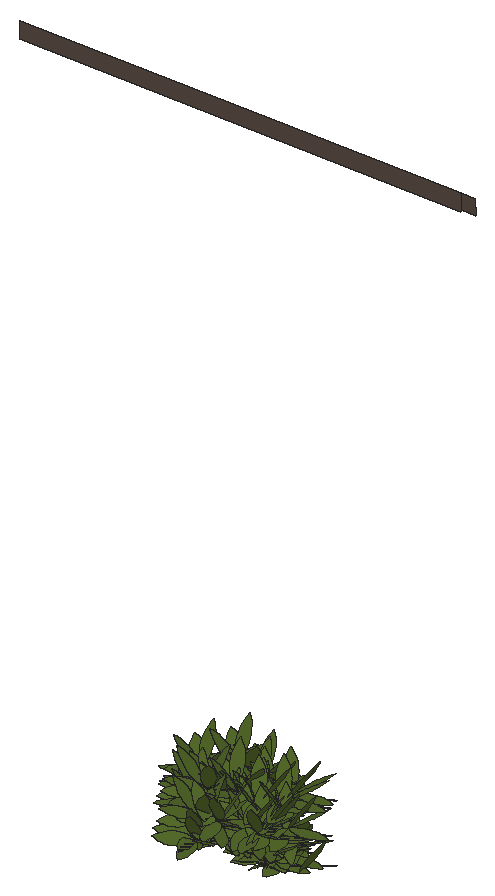
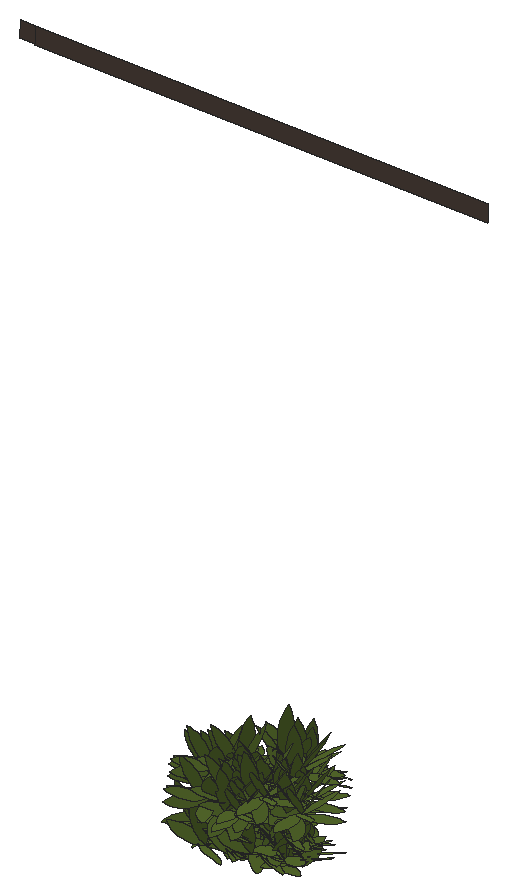
# SketchUp Ruby script. Lengths in inches.
U = 1.inch
M = Sketchup.active_model
def pt(a) = Geom::Point3d.new(a.map { |v| v * U })
def face(e, loops, mat)
  f = e.add_face(loops[0].map { |a| pt(a) })
  loops[1..].each { |l| e.add_face(l.map { |a| pt(a) }).erase! }
  f.material = f.back_material = mat if mat
  f
end
# faces: each face lists its corners as indices into pts; further lists are holes
def faces(e, pts, list, mat = nil) = list.each { |f| face(e, (f[0].is_a?(Array) ? f : [f]).map { |l| l.map { |i| pts[i] } }, mat) }
# xy, xz, yz: faces in a plane at the given z, y or x. An outline is a flat list of corners, or four numbers for a rectangle; further outlines are holes
def ring(l) = l.size == 4 ? [[l[0], l[1]], [l[2], l[1]], [l[2], l[3]], [l[0], l[3]]] : l.each_slice(2).to_a
def flat(e, list, mat, &to3) = list.each { |f| face(e, (f[0].is_a?(Array) ? f : [f]).map { |l| ring(l).map { |u, v| to3.(u, v) } }, mat) }
def xy(e, z, list, mat = nil) = flat(e, list, mat) { |x, y| [x, y, z] }
def xz(e, y, list, mat = nil) = flat(e, list, mat) { |x, z| [x, y, z] }
def yz(e, x, list, mat = nil) = flat(e, list, mat) { |y, z| [x, y, z] }
def lines(e, pts, list) = list.each { |a, b| e.add_line(pt(pts[a]), pt(pts[b])) }
# prism: a flat outline (further loops are holes) pulled along v
def prism(e, loops, v, mat = nil)
  f = face(e, loops, mat); d = Geom::Vector3d.new(v.map { |x| x * U })
  f.pushpull(f.normal.samedirection?(d) ? d.length : -d.length)
end
def box(e, o, s, mat = nil) = prism(e, [[o, [o[0] + s[0], o[1], o[2]], [o[0] + s[0], o[1] + s[1], o[2]], [o[0], o[1] + s[1], o[2]]]], [0, 0, s[2]], mat)
def at(x, y, z, deg = 0) = Geom::Transformation.translation(pt([x, y, z])) * Geom::Transformation.rotation(ORIGIN, Z_AXIS, deg.degrees)
def axes(o, x, y, z) = Geom::Transformation.new([*x, 0, *y, 0, *z, 0, *pt(o).to_a, 1])
def part(name) = M.definitions.add(name)
# library, detail: a bought-in or finely detailed component or shape, given as its bounding box
def library(name, o, s) = part(name).tap { |d| box(d.entities, o, s) }
def detail(e, o, s) = box(e.add_group.entities, o, s)
def put(e, d, t, mat = nil) = e.add_instance(d, t).tap { |i| i.material = mat if mat }
def group(e, t, mat = nil) = e.add_group.tap { |g| g.transformation = t; g.material = mat if mat }.entities
root = M.entities
M.materials.add("2").color = [91, 76, 69]
M.materials.add("[Asphalt_New]").color = [85, 106, 44]
M.materials.add("white").color = [255, 255, 255]
c1 = part("Component\#59")
xy(c1.entities,0,[[5.79,0,4.75,0.06,3.73,0.22,2.73,0.5,1.77,0.88,0.86,1.37,0,1.95,0.83,2.59,1.74,3.13,2.7,3.56,3.7,3.87,4.74,4.05,5.79,4.12,6.84,4.05,7.87,3.87,8.88,3.56,9.84,3.13,10.74,2.59,11.57,1.95,10.72,1.37,9.8,0.88,8.84,0.5,7.84,0.22,6.82,0.06]],"[Asphalt_New]")
c2 = part("Leaf cluster")
put(c2.entities,c1,axes([10.37,9.23,1.73],[-0.67725,-0.67301,0.29729],[0.61625,-0.73963,-0.27052],[0.40195,0,0.91566]),"[Asphalt_New]")
put(c2.entities,c1,at(0,5.84,1.2),"[Asphalt_New]")
put(c2.entities,c1,axes([11.625,9.72,1.52],[-0.61694,-0.11161,0.77906],[-0.02647,-0.98639,-0.16227],[0.78657,-0.12073,0.60559]),"[Asphalt_New]")
put(c2.entities,c1,axes([13.35,8.05,1.98],[-0.1211,0.99122,-0.05316],[-0.90762,-0.13226,-0.39842],[-0.40195,0,0.91566]),"[Asphalt_New]")
c3 = part("Groupe\#6")
put(c3.entities,c2,axes([6.2,8.72,2.56],[0.20072,0.20931,0],[-0.20931,0.20072,0],[0,0,0.3393]))
put(c3.entities,c2,axes([3.21,14.77,2.82],[0.12393,-0.26218,0],[0.26218,0.12393,0],[0,0,0.3393]))
put(c3.entities,c1,axes([6.98,12.58,2.74],[0.18147,-0.01125,0.26433],[0.07569,0.27597,-0.05506],[-0.21317,0.08841,0.20548]),"[Asphalt_New]")
put(c3.entities,c2,axes([9.62,7.71,2.12],[0.13301,0.2577,0],[-0.2577,0.13301,0],[0,0,0.3393]))
put(c3.entities,c2,axes([5.04,12.65,2.375],[0.19329,-0.21619,0],[0.21619,0.19329,0],[0,0,0.3393]))
put(c3.entities,c2,axes([8.55,8.27,2.12],[0.13301,0.2577,0],[-0.2577,0.13301,0],[0,0,0.3393]))
put(c3.entities,c2,axes([3.97,13.21,2.375],[0.19329,-0.21619,0],[0.21619,0.19329,0],[0,0,0.3393]))
put(c3.entities,c2,axes([13.2,6.93,2.95],[-0.24238,0.15922,0],[-0.15922,-0.24238,0],[0,0,0.3393]))
put(c3.entities,c2,axes([7.8,2.89,3.21],[0.23521,0.16964,0],[-0.16964,0.23521,0],[0,0,0.3393]))
put(c3.entities,c1,axes([9.26,7,3.13],[-0.02201,0.18048,0.26433],[-0.28514,0.02413,-0.05506],[-0.04808,-0.22571,0.20548]),"[Asphalt_New]")
put(c3.entities,c2,axes([10.92,8.49,3.88],[-0.24238,0.15922,0],[-0.15922,-0.24238,0],[0,0,0.3393]))
put(c3.entities,c2,axes([5.52,4.45,4.14],[0.23521,0.16964,0],[-0.16964,0.23521,0],[0,0,0.3393]))
put(c3.entities,c1,axes([6.97,8.56,4.0625],[-0.02201,0.18048,0.26433],[-0.28514,0.02413,-0.05506],[-0.04808,-0.22571,0.20548]),"[Asphalt_New]")
put(c3.entities,c2,axes([9.9,10.06,2.52],[-0.24238,0.15922,0],[-0.15922,-0.24238,0],[0,0,0.3393]))
put(c3.entities,c2,axes([4.51,6.02,2.78],[0.23521,0.16964,0],[-0.16964,0.23521,0],[0,0,0.3393]))
put(c3.entities,c1,axes([5.96,10.125,2.71],[-0.02201,0.18048,0.26433],[-0.28514,0.02413,-0.05506],[-0.04808,-0.22571,0.20548]),"[Asphalt_New]")
put(c3.entities,c2,axes([13.6,14.86,2.41],[-0.24779,-0.15066,0],[0.15066,-0.24779,0],[0,0,0.3393]))
put(c3.entities,c2,axes([8.65,12.2,2.15],[0.22914,-0.17774,0],[0.17774,0.22914,0],[0,0,0.3393]))
put(c3.entities,c2,axes([14.35,15.81,2.41],[-0.24779,-0.15066,0],[0.15066,-0.24779,0],[0,0,0.3393]))
put(c3.entities,c2,axes([7.9,11.25,2.15],[0.22914,-0.17774,0],[0.17774,0.22914,0],[0,0,0.3393]))
put(c3.entities,c2,axes([-0.46,12.1,3.24],[0.12393,-0.26218,0],[0.26218,0.12393,0],[0,0,0.3393]))
put(c3.entities,c1,axes([3.31,9.91,3.17],[0.18147,-0.01125,0.26433],[0.07569,0.27597,-0.05506],[-0.21317,0.08841,0.20548]),"[Asphalt_New]")
put(c3.entities,c2,axes([4.47,8.01,3.91],[0.20072,0.20931,0],[-0.20931,0.20072,0],[0,0,0.3393]))
put(c3.entities,c2,axes([1.49,14.06,4.17],[0.12393,-0.26218,0],[0.26218,0.12393,0],[0,0,0.3393]))
put(c3.entities,c1,axes([5.26,11.88,4.1],[0.18147,-0.01125,0.26433],[0.07569,0.27597,-0.05506],[-0.21317,0.08841,0.20548]),"[Asphalt_New]")
put(c3.entities,c2,axes([6.85,4.1,2.54],[0.13301,0.2577,0],[-0.2577,0.13301,0],[0,0,0.3393]))
put(c3.entities,c2,axes([2.27,9.05,2.8],[0.19329,-0.21619,0],[0.21619,0.19329,0],[0,0,0.3393]))
put(c3.entities,c1,axes([6.51,8.03,2.73],[0.17719,0.04076,0.26433],[-0.00581,0.2861,-0.05506],[-0.2295,0.02423,0.20548]),"[Asphalt_New]")
put(c3.entities,c2,axes([4.86,14.63,2.58],[0.22914,-0.17774,0],[0.17774,0.22914,0],[0,0,0.3393]))
put(c3.entities,c2,axes([10.5625,18.23,2.83],[-0.24779,-0.15066,0],[0.15066,-0.24779,0],[0,0,0.3393]))
put(c3.entities,c1,axes([8.79,14.25,2.76],[0.00779,-0.18165,0.26433],[0.28237,-0.04643,-0.05506],[0.06564,0.22124,0.20548]),"[Asphalt_New]")
put(c3.entities,c2,axes([7.02,12.9,3.51],[0.22914,-0.17774,0],[0.17774,0.22914,0],[0,0,0.3393]))
put(c3.entities,c2,axes([12.72,16.5,3.76],[-0.24779,-0.15066,0],[0.15066,-0.24779,0],[0,0,0.3393]))
put(c3.entities,c1,axes([10.94,12.52,3.6875],[0.00779,-0.18165,0.26433],[0.28237,-0.04643,-0.05506],[0.06564,0.22124,0.20548]),"[Asphalt_New]")
put(c3.entities,c2,axes([5.98,10.15,2.19],[0.23521,0.16964,0],[-0.16964,0.23521,0],[0,0,0.3393]))
put(c3.entities,c2,axes([9.23,9.05,2.52],[-0.24238,0.15922,0],[-0.15922,-0.24238,0],[0,0,0.3393]))
put(c3.entities,c2,axes([3.84,5.01,2.78],[0.23521,0.16964,0],[-0.16964,0.23521,0],[0,0,0.3393]))
put(c3.entities,c1,axes([5.29,9.12,2.71],[-0.02201,0.18048,0.26433],[-0.28514,0.02413,-0.05506],[-0.04808,-0.22571,0.20548]),"[Asphalt_New]")
put(c3.entities,c2,axes([4.09,12.81,2.58],[0.23461,-0.17046,0],[0.17046,0.23461,0],[0,0,0.3393]))
put(c3.entities,c2,axes([9.68,16.59,2.83],[-0.24294,-0.15837,0],[0.15837,-0.24294,0],[0,0,0.3393]))
put(c3.entities,c1,axes([8.03,12.56,2.76],[0.01349,-0.18132,0.26433],[0.28368,-0.03753,-0.05506],[0.05866,0.22319,0.20548]),"[Asphalt_New]")
put(c3.entities,c2,axes([6.3,11.15,3.51],[0.23461,-0.17046,0],[0.17046,0.23461,0],[0,0,0.3393]))
put(c3.entities,c2,axes([11.89,14.93,3.76],[-0.24294,-0.15837,0],[0.15837,-0.24294,0],[0,0,0.3393]))
put(c3.entities,c1,axes([10.24,10.89,3.6875],[0.01349,-0.18132,0.26433],[0.28368,-0.03753,-0.05506],[0.05866,0.22319,0.20548]),"[Asphalt_New]")
put(c3.entities,c2,axes([11.75,13.77,2.17],[-0.145,-0.25115,0],[0.25115,-0.145,0],[0,0,0.3393]))
put(c3.entities,c2,axes([16.09,8.62,2.43],[-0.1829,0.22505,0],[-0.22505,-0.1829,0],[0,0,0.3393]))
put(c3.entities,c2,axes([10.33,11.4,3.1],[-0.145,-0.25115,0],[0.25115,-0.145,0],[0,0,0.3393]))
put(c3.entities,c2,axes([14.67,6.25,3.36],[-0.1829,0.22505,0],[-0.22505,-0.1829,0],[0,0,0.3393]))
put(c3.entities,c1,axes([10.48,7.46,3.28],[-0.17891,-0.03237,0.26433],[-0.00768,-0.28605,-0.05506],[0.2281,-0.03501,0.20548]),"[Asphalt_New]")
put(c3.entities,c2,axes([7.24,9.53,2.15],[0.23461,-0.17046,0],[0.17046,0.23461,0],[0,0,0.3393]))
put(c3.entities,c2,axes([12.82,13.3125,2.41],[-0.24294,-0.15837,0],[0.15837,-0.24294,0],[0,0,0.3393]))
put(c3.entities,c2,axes([7.96,10.51,2.15],[0.23461,-0.17046,0],[0.17046,0.23461,0],[0,0,0.3393]))
put(c3.entities,c2,axes([13.54,14.29,2.41],[-0.24294,-0.15837,0],[0.15837,-0.24294,0],[0,0,0.3393]))
put(c3.entities,c2,axes([10,6.52,1.96],[0.20072,0.20931,0],[-0.20931,0.20072,0],[0,0,0.3393]))
put(c3.entities,c2,axes([7.01,12.5625,2.22],[0.12393,-0.26218,0],[0.26218,0.12393,0],[0,0,0.3393]))
put(c3.entities,c2,axes([5.33,9.5625,2.56],[0.20072,0.20931,0],[-0.20931,0.20072,0],[0,0,0.3393]))
put(c3.entities,c2,axes([2.34,15.61,2.82],[0.12393,-0.26218,0],[0.26218,0.12393,0],[0,0,0.3393]))
put(c3.entities,c1,axes([6.12,13.43,2.74],[0.18147,-0.01125,0.26433],[0.07569,0.27597,-0.05506],[-0.21317,0.08841,0.20548]),"[Asphalt_New]")
put(c3.entities,c2,axes([13.16,5.15,2],[-0.1829,0.22505,0],[-0.22505,-0.1829,0],[0,0,0.3393]))
put(c3.entities,c2,axes([14.2,4.53,2],[-0.1829,0.22505,0],[-0.22505,-0.1829,0],[0,0,0.3393]))
put(c3.entities,c2,axes([8.17,6.54,3.47],[0.13301,0.2577,0],[-0.2577,0.13301,0],[0,0,0.3393]))
put(c3.entities,c2,axes([3.58,11.48,3.73],[0.19329,-0.21619,0],[0.21619,0.19329,0],[0,0,0.3393]))
put(c3.entities,c1,axes([7.82,10.46,3.66],[0.17719,0.04076,0.26433],[-0.00581,0.2861,-0.05506],[-0.2295,0.02423,0.20548]),"[Asphalt_New]")
put(c3.entities,c2,axes([2.52,6.05,2.98],[0.20072,0.20931,0],[-0.20931,0.20072,0],[0,0,0.3393]))
xz(root,18.35,[[127.1875,121.625,148.875,122.4375]],"2")
p = [[148.875,18.37,121.69],[148.875,18.35,122.4375],[149.5625,18.35,122.4375],[149.5625,18.37,121.69]]
faces(root,p,[[0,1,2,3]],"2")
put(root,c2,axes([137.9,16.39,91.26],[0.1271,-0.08349,0],[0.08349,0.1271,0],[0,0,0.17792]),"white")
put(root,c2,axes([140.13,17.43,90.54],[-0.12016,0.09321,0],[-0.09321,-0.12016,0],[0,0,0.17792]),"white")
put(root,c2,axes([138.78,17.14,90.66],[-0.10136,0.11337,0],[-0.11337,-0.10136,0],[0,0,0.17792]),"white")
put(root,c3,axes([132.83,13.8,90.97],[0.48162,-0.20742,0],[0.20742,0.48162,0],[0,0,0.52438]),"white")
put(root,c1,axes([139.62,16.72,90.71],[0.15184,-0.00221,-0.00946],[-0.00119,0.13948,-0.07089],[0.0083,0.06056,0.16292]),"[Asphalt_New]")
put(root,c1,axes([138.09,16.1,90.93],[0.01807,0.15078,-0.00946],[-0.13884,0.01339,-0.07089],[-0.05936,0.01458,0.16292]),"[Asphalt_New]")
put(root,c1,axes([139.68,17.45,91.36],[-0.09292,-0.02137,0.13861],[0.00305,-0.15002,-0.02887],[0.12035,-0.0127,0.10775]),"[Asphalt_New]")
put(root,c1,axes([140.15,16.21,90.46],[0.10299,0.10235,0.0529],[-0.09371,0.11248,-0.04813],[-0.06112,0,0.16292]),"[Asphalt_New]")
put(root,c1,axes([137.5625,16.64,90.39],[0.09382,0.01697,0.13861],[0.00402,0.15,-0.02887],[-0.11961,0.01836,0.10775]),"[Asphalt_New]")
put(root,c1,axes([141.55,16.16,91.68],[0.01807,0.15078,-0.00946],[-0.13884,0.01339,-0.07089],[-0.05936,0.01458,0.16292]),"[Asphalt_New]")
put(root,c1,axes([139.71,17.42,92.15],[-0.15155,-0.00971,-0.00946],[0.01213,-0.13895,-0.07089],[-0.00352,-0.06102,0.16292]),"[Asphalt_New]")
put(root,c1,axes([138.73,16.19,91.52],[0.00875,0.15182,0],[-0.15182,0.00875,0],[0,0,0.17792]),"[Asphalt_New]")
put(root,c1,axes([140.83,16.19,90.9],[0.01807,0.15078,-0.00946],[-0.13884,0.01339,-0.07089],[-0.05936,0.01458,0.16292]),"[Asphalt_New]")
put(root,c1,axes([140.34,17.93,90.71],[0.01842,-0.15074,-0.00946],[0.13802,0.02011,-0.07089],[0.06112,0,0.16292]),"[Asphalt_New]")
put(root,c1,axes([137.94,16.78,91.31],[0.1519,0.00716,0],[-0.00716,0.1519,0],[0,0,0.17792]),"[Asphalt_New]")
put(root,c2,axes([139.35,16.82,90.89],[-0.06499,0.13748,0],[-0.13748,-0.06499,0],[0,0,0.17792]),"white")
put(root,c1,axes([137.34,18,91.74],[0.01842,-0.15074,-0.00946],[0.13802,0.02011,-0.07089],[0.06112,0,0.16292]),"[Asphalt_New]")
put(root,c2,axes([140.68,15.61,90.54],[0.07604,0.1317,0],[-0.1317,0.07604,0],[0,0,0.17792]),"white")
put(root,c1,axes([138.6,17.52,90.89],[-0.15155,-0.00971,-0.00946],[0.01213,-0.13895,-0.07089],[-0.00352,-0.06102,0.16292]),"[Asphalt_New]")
put(root,c1,axes([136.46,18.11,91.1],[-0.0159,-0.15124,0],[0.15124,-0.0159,0],[0,0,0.17792]),"[Asphalt_New]")
put(root,c2,axes([137.14,15.54,90.67],[0.12994,0.079,0],[-0.079,0.12994,0],[0,0,0.17792]),"white")
put(root,c1,axes([137.17,17.94,90.88],[-0.12443,-0.07482,0.0529],[0.06418,-0.13158,-0.04813],[0.05936,-0.01458,0.16292]),"[Asphalt_New]")
put(root,c2,axes([142.28,17.75,90.54],[-0.12303,0.08939,0],[-0.08939,-0.12303,0],[0,0,0.17792]),"white")
put(root,c2,axes([137.68,15.68,91.56],[0.07604,0.1317,0],[-0.1317,0.07604,0],[0,0,0.17792]),"white")
put(root,c2,axes([136.99,18.93,90.75],[-0.10525,-0.10976,0],[0.10976,-0.10525,0],[0,0,0.17792]),"white")
put(root,c1,axes([138.99,17,90.71],[0.15184,-0.00221,-0.00946],[-0.00119,0.13948,-0.07089],[0.0083,0.06056,0.16292]),"[Asphalt_New]")
put(root,c1,axes([138.43,17.5625,90.85],[-0.09516,0.0059,0.13861],[-0.03969,-0.14471,-0.02887],[0.11178,-0.04636,0.10775]),"[Asphalt_New]")
put(root,c2,axes([142.13,17.77,90.32],[-0.12016,0.09321,0],[-0.09321,-0.12016,0],[0,0,0.17792]),"white")
put(root,c2,axes([141.08,19.04,91.39],[-0.12334,-0.08896,0],[0.08896,-0.12334,0],[0,0,0.17792]),"white")
put(root,c1,axes([138.3,17.8,91.61],[0.09625,-0.10871,0.0529],[0.11768,0.08708,-0.04813],[0.00352,0.06102,0.16292]),"[Asphalt_New]")
put(root,c2,axes([135.37,17.28,90.43],[0.09591,-0.11801,0],[0.11801,0.09591,0],[0,0,0.17792]),"white")
put(root,c2,axes([140.74,17.02,90.89],[-0.06499,0.13748,0],[-0.13748,-0.06499,0],[0,0,0.17792]),"white")
put(root,c1,axes([137.24,16.8,91.16],[-0.00707,0.09508,0.13861],[-0.14876,0.01968,-0.02887],[-0.03076,-0.11704,0.10775]),"[Asphalt_New]")
put(root,c1,axes([137.04,16.58,91.2],[0.10299,0.10235,0.0529],[-0.09371,0.11248,-0.04813],[-0.06112,0,0.16292]),"[Asphalt_New]")
put(root,c2,axes([139.89,17.86,90.75],[-0.12016,0.09321,0],[-0.09321,-0.12016,0],[0,0,0.17792]),"white")
put(root,c1,axes([138.24,17.99,91.58],[0.01154,-0.09464,0.13861],[0.14952,-0.01265,-0.02887],[0.02521,0.11836,0.10775]),"[Asphalt_New]")
put(root,c1,axes([138.5625,18.14,90.88],[-0.12443,-0.07482,0.0529],[0.06418,-0.13158,-0.04813],[0.05936,-0.01458,0.16292]),"[Asphalt_New]")
put(root,c2,axes([139.35,15.77,90.67],[0.12739,0.08305,0],[-0.08305,0.12739,0],[0,0,0.17792]),"white")
put(root,c1,axes([136.77,16.59,90.93],[0.01807,0.15078,-0.00946],[-0.13884,0.01339,-0.07089],[-0.05936,0.01458,0.16292]),"[Asphalt_New]")
put(root,c2,axes([141.64,18,90.54],[-0.12303,0.08939,0],[-0.08939,-0.12303,0],[0,0,0.17792]),"white")
put(root,c2,axes([138.25,16.92,91.26],[0.1271,-0.08349,0],[0.08349,0.1271,0],[0,0,0.17792]),"white")
put(root,c1,axes([136.57,17.41,90.79],[0.14768,-0.03627,0],[0.03627,0.14768,0],[0,0,0.17792]),"[Asphalt_New]")
put(root,c1,axes([137.75,16.72,90.43],[0.10299,0.10235,0.0529],[-0.09371,0.11248,-0.04813],[-0.06112,0,0.16292]),"[Asphalt_New]")
put(root,c1,axes([139.91,16.95,90.63],[-0.00408,0.09525,0.13861],[-0.14807,0.02435,-0.02887],[-0.03442,-0.11602,0.10775]),"[Asphalt_New]")
put(root,c2,axes([139.14,15.88,90.46],[0.12994,0.079,0],[-0.079,0.12994,0],[0,0,0.17792]),"white")
put(root,c2,axes([139.74,17.29,90.67],[-0.06499,0.13748,0],[-0.13748,-0.06499,0],[0,0,0.17792]),"white")
put(root,c1,axes([141.6,17.22,90.42],[0.09382,0.01697,0.13861],[0.00402,0.15,-0.02887],[-0.11961,0.01836,0.10775]),"[Asphalt_New]")
put(root,c2,axes([140.2,19.33,92.11],[-0.12334,-0.08896,0],[0.08896,-0.12334,0],[0,0,0.17792]),"white")
put(root,c2,axes([141.62,18.11,90.54],[-0.12016,0.09321,0],[-0.09321,-0.12016,0],[0,0,0.17792]),"white")
put(root,c2,axes([138.93,17.81,90.66],[-0.10136,0.11337,0],[-0.11337,-0.10136,0],[0,0,0.17792]),"white")
put(root,c1,axes([141.97,17.97,90.36],[-0.15207,0,0],[0,-0.15207,0],[0,0,0.17792]),"[Asphalt_New]")
put(root,c1,axes([139.86,17.15,90.67],[-0.08742,0.11593,0.0529],[-0.12415,-0.07758,-0.04813],[-0.0083,-0.06056,0.16292]),"[Asphalt_New]")
put(root,c2,axes([136.9,15.98,90.89],[0.12994,0.079,0],[-0.079,0.12994,0],[0,0,0.17792]),"white")
put(root,c1,axes([137.79,17.4,90.71],[0.15184,-0.00221,-0.00946],[-0.00119,0.13948,-0.07089],[0.0083,0.06056,0.16292]),"[Asphalt_New]")
put(root,c2,axes([138.82,18.14,90.54],[-0.12016,0.09321,0],[-0.09321,-0.12016,0],[0,0,0.17792]),"white")
put(root,c1,axes([137.375,17.97,90.85],[-0.09516,0.0059,0.13861],[-0.03969,-0.14471,-0.02887],[0.11178,-0.04636,0.10775]),"[Asphalt_New]")
put(root,c1,axes([137.5625,18.41,90.67],[-0.12443,-0.07482,0.0529],[0.06418,-0.13158,-0.04813],[0.05936,-0.01458,0.16292]),"[Asphalt_New]")
put(root,c1,axes([136.84,18.62,91.1],[-0.0159,-0.15124,0],[0.15124,-0.0159,0],[0,0,0.17792]),"[Asphalt_New]")
put(root,c2,axes([138.71,16.02,90.67],[0.12739,0.08305,0],[-0.08305,0.12739,0],[0,0,0.17792]),"white")
put(root,c2,axes([139.1,19.43,90.84],[-0.12334,-0.08896,0],[0.08896,-0.12334,0],[0,0,0.17792]),"white")
put(root,c1,axes([138.125,18.58,91.02],[0.01842,-0.15074,-0.00946],[0.13802,0.02011,-0.07089],[0.06112,0,0.16292]),"[Asphalt_New]")
put(root,c1,axes([140.2,17.38,90.42],[0.09382,0.01697,0.13861],[0.00402,0.15,-0.02887],[-0.11961,0.01836,0.10775]),"[Asphalt_New]")
put(root,c2,axes([137.37,17.21,91.97],[0.1271,-0.08349,0],[0.08349,0.1271,0],[0,0,0.17792]),"white")
put(root,c2,axes([138.8,19.34,90.49],[-0.06975,-0.13513,0],[0.13513,-0.06975,0],[0,0,0.17792]),"white")
put(root,c2,axes([138.47,16.26,90.85],[0.07604,0.1317,0],[-0.1317,0.07604,0],[0,0,0.17792]),"white")
put(root,c1,axes([139.27,17.22,90.63],[-0.00408,0.09525,0.13861],[-0.14807,0.02435,-0.02887],[-0.03442,-0.11602,0.10775]),"[Asphalt_New]")
put(root,c1,axes([139.25,17.04,90.67],[-0.0255,0.1497,-0.00946],[-0.13692,-0.02659,-0.07089],[-0.06106,-0.00288,0.16292]),"[Asphalt_New]")
put(root,c2,axes([140.43,18.37,90.54],[-0.12303,0.08939,0],[-0.08939,-0.12303,0],[0,0,0.17792]),"white")
put(root,c1,axes([139.5625,18.78,90.58],[-0.02064,-0.15066,0],[0.15066,-0.02064,0],[0,0,0.17792]),"[Asphalt_New]")
put(root,c2,axes([136.27,17.3125,90.71],[0.1271,-0.08349,0],[0.08349,0.1271,0],[0,0,0.17792]),"white")
put(root,c1,axes([138.51,18.24,91.66],[-0.15155,-0.00971,-0.00946],[0.01213,-0.13895,-0.07089],[-0.00352,-0.06102,0.16292]),"[Asphalt_New]")
put(root,c1,axes([138.76,18.16,90.85],[-0.09516,0.0059,0.13861],[-0.03969,-0.14471,-0.02887],[0.11178,-0.04636,0.10775]),"[Asphalt_New]")
put(root,c2,axes([138.63,16.22,90.67],[0.12994,0.079,0],[-0.079,0.12994,0],[0,0,0.17792]),"white")
put(root,c2,axes([138.84,19.59,90.75],[-0.10525,-0.10976,0],[0.10976,-0.10525,0],[0,0,0.17792]),"white")
put(root,c2,axes([139.4,17.86,90.46],[0.09591,-0.11801,0],[0.11801,0.09591,0],[0,0,0.17792]),"white")
put(root,c1,axes([139.23,17.42,90.67],[-0.08742,0.11593,0.0529],[-0.12415,-0.07758,-0.04813],[-0.0083,-0.06056,0.16292]),"[Asphalt_New]")
put(root,c1,axes([139.9375,17.65,90.71],[0.15183,0.00256,-0.00946],[-0.00557,0.13937,-0.07089],[0.00639,0.06079,0.16292]),"[Asphalt_New]")
put(root,c1,axes([142.37,18.27,90.58],[-0.15207,0,0],[0,-0.15207,0],[0,0,0.17792]),"[Asphalt_New]")
put(root,c2,axes([139.5,19.51,91.27],[-0.06975,-0.13513,0],[0.13513,-0.06975,0],[0,0,0.17792]),"white")
put(root,c1,axes([139.78,17.75,90.5],[0.15184,-0.00221,-0.00946],[-0.00119,0.13948,-0.07089],[0.0083,0.06056,0.16292]),"[Asphalt_New]")
put(root,c1,axes([139.95,17.21,91.45],[-0.0255,0.1497,-0.00946],[-0.13692,-0.02659,-0.07089],[-0.06106,-0.00288,0.16292]),"[Asphalt_New]")
put(root,c1,axes([139.37,18.34,91.6],[-0.15207,0,0],[0,-0.15207,0],[0,0,0.17792]),"[Asphalt_New]")
put(root,c1,axes([137.58,18.9,91.02],[0.01842,-0.15074,-0.00946],[0.13802,0.02011,-0.07089],[0.06112,0,0.16292]),"[Asphalt_New]")
put(root,c2,axes([137.5,16.39,90.67],[0.12739,0.08305,0],[-0.08305,0.12739,0],[0,0,0.17792]),"white")
put(root,c1,axes([140.6,17.68,90.63],[0.09382,0.01697,0.13861],[0.00402,0.15,-0.02887],[-0.11961,0.01836,0.10775]),"[Asphalt_New]")
put(root,c2,axes([138.01,18.02,90.46],[0.09591,-0.11801,0],[0.11801,0.09591,0],[0,0,0.17792]),"white")
put(root,c1,axes([136.91,18.01,90.79],[0.14768,-0.03627,0],[0.03627,0.14768,0],[0,0,0.17792]),"[Asphalt_New]")
put(root,c1,axes([137.55,17.84,90.93],[0.15184,-0.00221,-0.00946],[-0.00119,0.13948,-0.07089],[0.0083,0.06056,0.16292]),"[Asphalt_New]")
put(root,c1,axes([138.93,19.05,90.58],[-0.02064,-0.15066,0],[0.15066,-0.02064,0],[0,0,0.17792]),"[Asphalt_New]")
put(root,c2,axes([137.92,16.58,90.85],[0.07604,0.1317,0],[-0.1317,0.07604,0],[0,0,0.17792]),"white")
put(root,c1,axes([138.62,17.25,90.93],[0.01807,0.15078,-0.00946],[-0.13884,0.01339,-0.07089],[-0.05936,0.01458,0.16292]),"[Asphalt_New]")
put(root,c1,axes([137.6,17.75,91.65],[0.09382,0.01697,0.13861],[0.00402,0.15,-0.02887],[-0.11961,0.01836,0.10775]),"[Asphalt_New]")
put(root,c1,axes([137.77,18.43,90.63],[-0.09516,0.0059,0.13861],[-0.03969,-0.14471,-0.02887],[0.11178,-0.04636,0.10775]),"[Asphalt_New]")
put(root,c1,axes([140.47,19.03,90.5],[0.01842,-0.15074,-0.00946],[0.13802,0.02011,-0.07089],[0.06112,0,0.16292]),"[Asphalt_New]")
put(root,c1,axes([139.3,17.9,90.71],[0.15183,0.00256,-0.00946],[-0.00557,0.13937,-0.07089],[0.00639,0.06079,0.16292]),"[Asphalt_New]")
put(root,c2,axes([136.375,19.73,90.52],[-0.06975,-0.13513,0],[0.13513,-0.06975,0],[0,0,0.17792]),"white")
put(root,c1,axes([138.07,17.63,90.63],[-0.00408,0.09525,0.13861],[-0.14807,0.02435,-0.02887],[-0.03442,-0.11602,0.10775]),"[Asphalt_New]")
put(root,c2,axes([142.41,18.77,90.32],[-0.12303,0.08939,0],[-0.08939,-0.12303,0],[0,0,0.17792]),"white")
put(root,c2,axes([140.8125,16.71,90.32],[0.07604,0.1317,0],[-0.1317,0.07604,0],[0,0,0.17792]),"white")
put(root,c1,axes([140.39,17.46,90.46],[0.10299,0.10235,0.0529],[-0.09371,0.11248,-0.04813],[-0.06112,0,0.16292]),"[Asphalt_New]")
put(root,c2,axes([140.17,18.8,90.75],[-0.12303,0.08939,0],[-0.08939,-0.12303,0],[0,0,0.17792]),"white")
put(root,c2,axes([137.79,19.99,90.75],[-0.10525,-0.10976,0],[0.10976,-0.10525,0],[0,0,0.17792]),"white")
put(root,c2,axes([140.48,18.79,90.54],[-0.12016,0.09321,0],[-0.09321,-0.12016,0],[0,0,0.17792]),"white")
put(root,c1,axes([138.03,17.83,90.67],[-0.08742,0.11593,0.0529],[-0.12415,-0.07758,-0.04813],[-0.0083,-0.06056,0.16292]),"[Asphalt_New]")
put(root,c1,axes([139.28,18.08,90.71],[0.15184,-0.00221,-0.00946],[-0.00119,0.13948,-0.07089],[0.0083,0.06056,0.16292]),"[Asphalt_New]")
put(root,c1,axes([135.91,18.28,90.58],[0.14768,-0.03627,0],[0.03627,0.14768,0],[0,0,0.17792]),"[Asphalt_New]")
